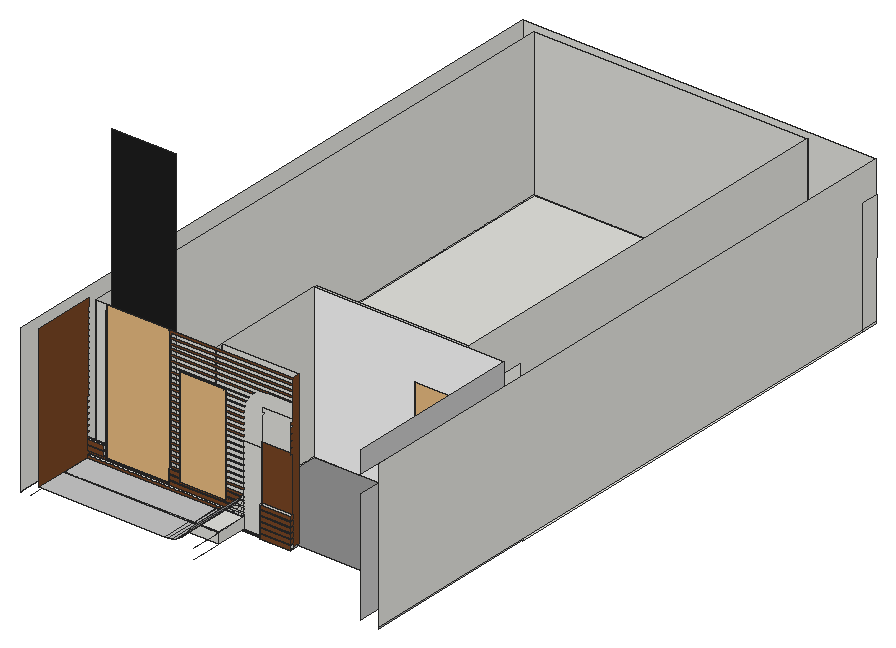
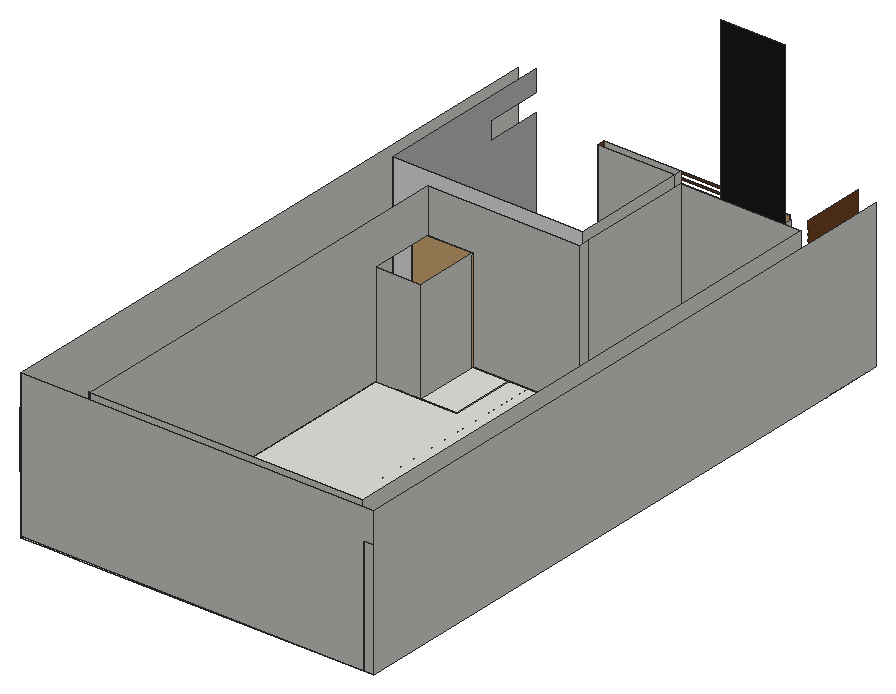
# SketchUp Ruby script. Lengths in inches.
U = 1.inch
M = Sketchup.active_model
def pt(a) = Geom::Point3d.new(a.map { |v| v * U })
def face(e, loops, mat)
  f = e.add_face(loops[0].map { |a| pt(a) })
  loops[1..].each { |l| e.add_face(l.map { |a| pt(a) }).erase! }
  f.material = f.back_material = mat if mat
  f
end
# faces: each face lists its corners as indices into pts; further lists are holes
def faces(e, pts, list, mat = nil) = list.each { |f| face(e, (f[0].is_a?(Array) ? f : [f]).map { |l| l.map { |i| pts[i] } }, mat) }
# xy, xz, yz: faces in a plane at the given z, y or x. An outline is a flat list of corners, or four numbers for a rectangle; further outlines are holes
def ring(l) = l.size == 4 ? [[l[0], l[1]], [l[2], l[1]], [l[2], l[3]], [l[0], l[3]]] : l.each_slice(2).to_a
def flat(e, list, mat, &to3) = list.each { |f| face(e, (f[0].is_a?(Array) ? f : [f]).map { |l| ring(l).map { |u, v| to3.(u, v) } }, mat) }
def xy(e, z, list, mat = nil) = flat(e, list, mat) { |x, y| [x, y, z] }
def xz(e, y, list, mat = nil) = flat(e, list, mat) { |x, z| [x, y, z] }
def yz(e, x, list, mat = nil) = flat(e, list, mat) { |y, z| [x, y, z] }
def lines(e, pts, list) = list.each { |a, b| e.add_line(pt(pts[a]), pt(pts[b])) }
# prism: a flat outline (further loops are holes) pulled along v
def prism(e, loops, v, mat = nil)
  f = face(e, loops, mat); d = Geom::Vector3d.new(v.map { |x| x * U })
  f.pushpull(f.normal.samedirection?(d) ? d.length : -d.length)
end
def box(e, o, s, mat = nil) = prism(e, [[o, [o[0] + s[0], o[1], o[2]], [o[0] + s[0], o[1] + s[1], o[2]], [o[0], o[1] + s[1], o[2]]]], [0, 0, s[2]], mat)
def at(x, y, z, deg = 0) = Geom::Transformation.translation(pt([x, y, z])) * Geom::Transformation.rotation(ORIGIN, Z_AXIS, deg.degrees)
def axes(o, x, y, z) = Geom::Transformation.new([*x, 0, *y, 0, *z, 0, *pt(o).to_a, 1])
def part(name) = M.definitions.add(name)
# library, detail: a bought-in or finely detailed component or shape, given as its bounding box
def library(name, o, s) = part(name).tap { |d| box(d.entities, o, s) }
def detail(e, o, s) = box(e.add_group.entities, o, s)
def put(e, d, t, mat = nil) = e.add_instance(d, t).tap { |i| i.material = mat if mat }
def group(e, t, mat = nil) = e.add_group.tap { |g| g.transformation = t; g.material = mat if mat }.entities
root = M.entities
M.materials.add("Moss 1").color = [97, 97, 43]
M.materials.add("[Color M00]").color = [255, 255, 255]
M.materials.add("[Color M02]").color = [198, 198, 198]
M.materials.add("[Color M03]").color = [170, 170, 170]
M.materials.add("[Color M04]1").color = [142, 142, 142]
M.materials.add("[Color M08]1").color = [30, 30, 30]
M.materials.add("[Groundcover_Wood_Mix]").color = [133, 121, 115]
M.materials.add("[Wood Veneer 01]").color = [120, 70, 37]
c1 = part("HCD  9x9 Indo Pot (Square)")
xy(c1.entities,0,[[0,0,9,9]])
xy(c1.entities,0.75,[[0.75,0.75,8.25,8.25]])
xy(c1.entities,7.52,[[0.75,0.75,8.25,8.25]],"Moss 1")
xy(c1.entities,9,[[[0,0,9,9],[0.75,0.75,8.25,8.25]]])
xz(c1.entities,0,[[0,0,9,9]])
xz(c1.entities,0.75,[[0.75,0.75,8.25,7.52],[0.75,7.52,8.25,9]])
xz(c1.entities,8.25,[[0.75,0.75,8.25,7.52],[0.75,7.52,8.25,9]])
xz(c1.entities,9,[[0,0,9,9]])
yz(c1.entities,0,[[0,0,9,9]])
yz(c1.entities,0.75,[[0.75,0.75,8.25,7.52],[0.75,7.52,8.25,9]])
yz(c1.entities,8.25,[[0.75,0.75,8.25,7.52],[0.75,7.52,8.25,9]])
yz(c1.entities,9,[[0,0,9,9]])
c2 = part("Group\#284")
detail(c2.entities,[0,0,0],[2.15,3.79,14.3])
c3 = part("Potted plant")
put(c3.entities,c1,axes([7.375,7.93,0],[1.35,0,0],[0,1.35,0],[0,0,1.35]))
g1 = group(c3.entities,at(34.01,16.59,10.48),"[Groundcover_Wood_Mix]")
put(g1,c2,axes([-21.39,-3.67,0.04],[1.0831,1.67432,0],[1.44561,-0.94233,-0.44822],[0.5095,-0.33212,1.35364]))
put(g1,c2,axes([-19.2,-0.0625,0.04],[0.06577,-1.58752,0],[-1.23,-0.01362,-0.59477],[-0.71488,-0.00792,0.95418]))
put(g1,c2,axes([-20.16,-2.02,1.03],[1.23757,0.97175,0],[0.71987,-0.88743,-0.73204],[0.35645,-0.43942,0.56976]))
put(g1,c2,axes([-20.43,-4.53,0.04],[0.02652,1.58591,0],[1.23087,-0.05659,-0.59477],[0.71539,-0.03289,0.95418]))
put(g1,c2,axes([-19.73,-2.8125,1.03],[-1.55944,0.41251,0],[0.26154,1.08365,-0.73204],[0.12951,0.53658,0.56976]))
put(g1,c2,axes([-19.27,-4.42,0.04],[-1.00701,1.78126,0],[1.48381,0.79245,-0.44822],[0.52297,0.2793,1.35364]))
put(g1,c2,axes([-17.53,-1.6,0.04],[-1.30559,-0.8818,0],[-0.71402,1.01403,-0.59477],[-0.41499,0.58936,0.95418]))
put(g1,c2,axes([-21.8,-1.55,0.04],[2.03404,-0.13573,0],[-0.064,-1.68745,-0.44822],[-0.02256,-0.59474,1.35364]))
put(g1,c2,axes([-19.33,-2.61,1.03],[-1.22683,-0.98484,0],[-0.72899,0.88019,-0.73204],[-0.36097,0.43583,0.56976]))
put(g1,c2,axes([-19.3,-2.11,1.03],[0.27974,-1.57083,0],[-1.11549,-0.16277,-0.73204],[-0.55235,-0.0806,0.56976]))
put(g1,c2,axes([-21.97,-3.02,0.04],[1.31205,0.87256,0],[0.70701,-1.01874,-0.59477],[0.41092,-0.59209,0.95418]))
put(g1,c2,axes([-17.81,-3.69,0.04],[-1.51859,0.55236,0],[0.39363,1.14324,-0.59477],[0.22878,0.66446,0.95418]))
put(g1,c2,axes([-20.2,-2.52,1.03],[-0.299,1.5679,0],[1.11299,0.17632,-0.73204],[0.55111,0.08731,0.56976]))
put(g1,c2,axes([-21.28,-0.49,0.04],[1.33266,-0.92103,0],[-0.68389,-0.99325,-0.59477],[-0.39748,-0.57728,0.95418]))
put(g1,c2,axes([-19.17,-0.27,0.04],[-0.5456,-1.92548,0],[1.93945,-0.59168,-0.26656],[0.28985,-0.08843,1.78359]))
put(g1,c2,axes([-17.96,-1.15,0.04],[-1.27123,-1.53638,0],[-1.33347,1.09526,-0.44822],[-0.46998,0.38602,1.35364]))
put(g1,c2,axes([-19.65,-1.83,1.03],[1.43123,-0.75657,0],[-0.50987,-0.98658,-0.73204],[-0.25247,-0.48851,0.56976]))
put(g1,c2,axes([-16.8,-2.55,0.04],[-1.5632,-0.30402,0],[0.34989,-1.54112,-0.20989],[0.05229,-0.23032,1.4044]))
put(g1,c2,axes([-21.84,-2.79,0.04],[1.97107,0.44464,0],[-0.50241,1.94504,-0.26656],[-0.07509,0.29069,1.78359]))
put(g1,c2,axes([-20.37,0.56,0.04],[0.7463,-1.42646,0],[1.4028,0.68931,-0.20989],[0.20965,0.10302,1.4044]))
put(g1,c2,axes([-17.99,-3.6,0.04],[-1.66024,1.21511,0],[-1.16467,-1.59132,-0.26656],[-0.17406,-0.23783,1.78359]))
put(g1,c2,axes([-21.54,-4.58,0.04],[0.59386,1.45638,0],[-1.47231,0.6251,-0.20989],[-0.22004,0.09342,1.4044]))
put(g1,c2,axes([-19.92,-0.17,0.04],[0.74111,-1.89898,0],[-1.5902,-0.56846,-0.44822],[-0.56047,-0.20035,1.35364]))
c4 = library("door (1)",[38.93,25.48,0],[40,9.94,82.68])
c5 = library("Group\#414",[0,0,0],[35.43,0.39,70.87])
xy(root,60.3,[[480.01,345.98,505.26,349.54]],"[Wood Veneer 01]")
xy(root,60.625,[[338.49,355.04,437.21,449.29],[441.95,355.04,480.01,449.29],[480.01,355.04,561.55,449.29],[338.49,449.29,338.49,804.16,480.01,804.16,480.01,458.23,437.21,458.23,437.21,449.29],[480.01,449.29,495.24,458.23],
  [543.24,449.29,568.49,449.29,568.49,811.1,480.01,811.1,480.01,804.16,561.55,804.16,561.55,458.23,543.24,458.23],[495.24,449.29,543.24,458.23],[480.01,458.23,495.24,458.23,495.24,511.73,543.24,511.73,543.24,458.23,561.55,458.23,561.55,804.16,480.01,804.16],[495.24,458.23,543.24,511.73],[495.24,458.23,543.24,511.73]])
xy(root,60.75,[[480.01,345.98,505.26,348.1]])
xy(root,61.72,[[338.58,322.42,338.63,348.1],[338.63,322.42,465.45,348.1]])
xy(root,61.75,[[612.67,301.92,612.67,348.42,612.66,348.42,612.66,449.29,574.17,449.29,574.17,458.23,568.49,458.23,568.49,811.1,612.68,811.1,612.68,301.92],[323.43,348.42,331.5,449.29],[331.5,348.42,331.55,449.29],[331.55,348.42,346.7,348.42,346.7,355.04,338.49,355.04,338.49,449.29,331.55,449.29],[346.7,348.42,441.95,348.42,441.95,449.29,437.21,449.29,437.21,355.04,346.7,355.04],
  [441.95,348.42,480.01,355.04],[480.01,348.42,505.26,355.04],[338.49,355.04,346.7,449.29],[346.7,355.04,437.21,449.29],[323.43,449.29,331.55,811.1],
  [338.49,449.29,437.21,449.29,437.21,458.23,495.24,458.23,495.24,511.73,561.55,511.73,561.55,804.16,338.49,804.16],[495.24,449.29,524.68,458.23],[524.68,449.29,574.17,458.23],[495.24,458.23,524.68,511.73],[524.68,458.23,543.24,511.73],
  [543.24,458.23,561.55,511.73],[561.55,458.23,562.67,804.16]])
xy(root,61.75,[[612.66,301.92,612.67,348.42],[480.01,346.79,505.26,348.42]],"[Color M03]")
xy(root,61.75,[[505.26,352.35,597.79,352.35,597.79,449.29,441.95,449.29,441.95,355.04,505.26,355.04]],"[Color M04]1")
xy(root,63.8,[[480.01,345.98,505.26,348.1]])
xy(root,65.14,[[480.01,345.98,505.26,348.1]],"[Wood Veneer 01]")
xy(root,68.1875,[[480.01,345.98,505.26,348.1]])
xy(root,69.52,[[480.01,345.98,505.26,348.1]],"[Wood Veneer 01]")
xy(root,70.22,[[441.44,322.42,465.45,348.1]])
xy(root,70.22,[[338.58,296.73,441.44,322.42]],"[Color M02]")
xy(root,70.42,[[444.57,322.42,465.45,348.1],[338.58,345.98,444.57,348.1]])
xy(root,70.42,[[338.58,322.42,444.57,345.98]],"[Color M02]")
xy(root,72.57,[[338.58,345.98,451.7,348.1],[480.01,345.98,505.26,348.1]])
xy(root,73.68,[[352.5,348.1,404.9375,354.42]])
xy(root,73.91,[[405.46,345.98,454.16,348.1]])
xy(root,73.91,[[480.01,345.98,505.26,348.1]],"[Wood Veneer 01]")
xy(root,75.875,[[338.58,345.98,352.5,348.1]])
xy(root,76.96,[[405.46,345.98,458.09,348.1],[480.01,345.98,505.26,348.1]])
xy(root,78.29,[[405.46,345.98,459.33,348.1],[480.01,345.98,505.26,348.1]])
xy(root,79.59,[[338.58,345.98,352.5,348.1]])
xy(root,80.25,[[338.58,345.98,352.5,348.1]])
xy(root,81.34,[[405.46,345.98,461.65,348.1],[480.01,345.98,505.26,348.1]])
xy(root,82.68,[[405.46,345.98,462.46,348.1],[480.01,345.98,505.26,348.1]])
xy(root,83.97,[[338.58,345.98,352.5,348.1]])
xz(root,322.42,[[338.58,61.72,465.45,70.22],[338.58,70.22,465.45,70.42]])
xz(root,345.98,[[419.16,81.34,450.71,82.68]])
xz(root,345.98,[[480.01,60.75,505.26,63.8],[480.01,65.14,505.26,68.1875],[480.01,69.52,505.26,72.57],[338.58,70.42,444.57,70.42,447.66,71.03,450.63,72.04,451.7,72.57,338.58,72.57],[405.46,73.91,454.16,73.91,456.06,75.18,458.09,76.96,405.46,76.96],
  [480.01,73.91,505.26,76.96],[338.58,75.875,352.5,79.59],[405.46,78.29,419.16,81.34],[419.16,78.29,450.71,81.34],[450.71,78.29,459.33,78.29,460.49,79.61,461.65,81.34,450.71,81.34],
  [480.01,78.29,505.26,81.34],[338.58,80.25,352.5,83.97],[405.46,82.68,419.16,85.73],[419.16,82.68,450.71,85.73],[450.71,82.68,462.46,82.68,463.625,85.04,463.86,85.73,450.71,85.73],
  [480.01,82.68,505.26,85.73]],"[Wood Veneer 01]")
xz(root,348.1,[[405.46,60.75,405.46,61.4,454.2,61.17,454.78,61.16,454.16,60.75],[454.16,60.75,454.78,61.16,459.68,61.14,459.33,60.75],[459.33,60.75,459.68,61.14,462.65,61.125,462.46,60.75],[462.46,60.75,462.65,61.125,464.4375,61.12,464.3125,60.75],[464.3125,60.75,464.4375,61.12,465.3,61.11,465.27,60.75],
  [465.27,60.75,465.3,61.11,465.45,61.11,465.45,60.75],[480.01,61.04,480.01,61.11,465.45,61.11],[465.3,61.11,465.3,61.17,464.45,61.17,464.4375,61.12],[465.3,61.11,465.45,61.17],[465.45,61.11,480.01,61.17],
  [464.4375,61.12,464.45,61.17,462.67,61.17,462.65,61.125],[462.65,61.125,462.67,61.17,459.7,61.17,459.68,61.14],[459.68,61.14,459.7,61.17,454.78,61.17,454.78,61.16],[454.78,61.16,454.78,61.17,454.2,61.17],[454.2,61.17,454.78,61.17,455.2,61.44,441.44,61.44,444.57,61.65,455.5,61.65,455.6,61.72,405.46,61.72,405.46,61.4],
  [454.78,61.17,459.7,61.17,459.94,61.44,460.125,61.65,460.18,61.72,455.6,61.72,455.2,61.44],[459.7,61.17,462.67,61.17,462.8,61.44,462.9,61.65,462.9375,61.72,460.18,61.72,460.125,61.65,459.94,61.44],[462.67,61.17,464.45,61.17,464.55,61.44,464.62,61.65,464.64,61.7,464.64,61.72,462.9375,61.72,462.9,61.65,462.8,61.44],[464.45,61.17,465.3,61.17,465.32,61.44,465.33,61.65,465.33,61.72,464.64,61.72,464.64,61.7,464.62,61.65,464.55,61.44],[465.3,61.17,465.45,61.17,465.45,61.72,465.33,61.72,465.33,61.65,465.32,61.44],
  [465.45,61.17,480.01,61.72],[405.46,61.4,405.46,61.72,338.63,61.72,346.76,61.68],[441.44,61.44,455.2,61.44,455.5,61.65,444.57,61.65],[338.58,61.72,405.46,61.72,405.46,63.8,465.45,63.8,465.45,65.14,405.46,65.14,405.46,68.1875,465.45,68.1875,465.45,69.52,405.46,69.52,338.58,70.42],[405.46,61.72,455.6,61.72,456.06,62.02,458.09,63.8,405.46,63.8],
  [455.6,61.72,460.18,61.72,460.49,62.07,461.65,63.8,458.09,63.8,456.06,62.02],[460.18,61.72,462.9375,61.72,463.625,63.11,463.86,63.8,461.65,63.8,460.49,62.07],[462.9375,61.72,464.64,61.72,465.05,63.8,463.86,63.8,463.625,63.11],[464.64,61.72,465.33,61.72,465.45,63.53,465.45,63.8,465.05,63.8],[465.33,61.72,465.45,61.72,465.45,63.53],
  [465.45,61.72,480.01,126.53],[405.46,65.14,464.3125,65.14,464.55,65.83,464.62,66.04,464.64,66.09,465.05,68.1875,405.46,68.1875],[464.3125,65.14,465.27,65.14,465.32,65.83,465.33,66.04,465.45,67.92,465.45,68.1875,465.05,68.1875,464.64,66.09,464.62,66.04,464.55,65.83],[465.27,65.14,465.45,65.14,465.45,67.92,465.33,66.04,465.32,65.83],[480.01,65.14,505.26,68.1875],
  [441.44,65.83,455.2,65.83,455.5,66.04,444.57,66.04],[405.46,69.52,454.16,69.52,455.2,70.22,441.44,70.22,444.57,70.42,338.58,70.42],[454.16,69.52,459.33,69.52,459.94,70.22,455.2,70.22],[459.33,69.52,462.46,69.52,462.8,70.22,459.94,70.22],[462.46,69.52,464.3125,69.52,464.55,70.22,462.8,70.22],
  [464.3125,69.52,465.27,69.52,465.32,70.22,464.55,70.22],[465.27,69.52,465.45,69.52,465.45,70.22,465.32,70.22],[480.01,69.52,505.26,72.57],[441.44,70.22,455.2,70.22,455.5,70.42,444.57,70.42],[455.2,70.22,455.5,70.42,460.125,70.42,459.94,70.22],
  [459.94,70.22,460.125,70.42,462.9,70.42,462.8,70.22],[462.8,70.22,462.9,70.42,464.62,70.42,464.55,70.22],[464.55,70.22,464.62,70.42,465.33,70.42,465.32,70.22],[465.32,70.22,465.33,70.42,465.45,70.42,465.45,70.22],[338.58,70.42,338.58,72.57,451.7,72.57,450.63,72.04,447.66,71.03,444.57,70.42],
  [444.57,70.42,455.5,70.42,456.06,70.79,458.09,72.57,451.7,72.57,450.63,72.04,447.66,71.03],[405.46,73.91,405.46,76.96,458.09,76.96,456.06,75.18,454.16,73.91],[454.16,73.91,459.33,73.91,460.49,75.23,461.65,76.96,458.09,76.96,456.06,75.18],[480.01,73.91,505.26,76.96],[338.58,75.875,352.5,79.59],
  [405.46,78.29,405.46,81.34,461.65,81.34,460.49,79.61,459.33,78.29],[459.33,78.29,462.46,78.29,463.625,80.65,463.86,81.34,461.65,81.34,460.49,79.61],[480.01,78.29,505.26,81.34],[338.58,79.59,352.5,80.25],[338.58,80.25,352.5,83.97],
  [405.46,82.68,405.46,85.73,463.86,85.73,463.625,85.04,462.46,82.68],[462.46,82.68,464.3125,82.68,464.64,83.63,465.05,85.73,463.86,85.73,463.625,85.04],[480.01,82.68,505.26,85.73],[338.58,83.97,352.5,84.625]])
xz(root,348.1,[[480.01,60.75,505.26,63.8],[338.58,72.57,451.7,72.57,453.45,73.43,454.16,73.91,405.46,73.91,405.46,76.96,458.09,76.96,458.42,77.25,459.33,78.29,405.46,78.29,405.46,81.34,461.65,81.34,462.24,82.22,462.46,82.68,405.46,82.68,405.46,85.73,463.86,85.73,464.3125,87.0625,405.46,87.0625,405.46,90.11,465.05,90.11,465.25,91.1,465.27,91.45,405.46,91.45,405.46,94.5,465.45,94.5,465.45,95.83,405.46,95.83,405.46,98.88,465.45,98.88,465.45,100.22,405.46,100.22,405.46,103.27,465.45,103.27,465.45,104.6,405.46,104.6,405.46,107.66,465.45,107.66,465.45,108.99,405.46,108.99,405.46,112.04,465.45,112.04,465.45,113.375,405.46,113.375,405.46,116.43,465.45,116.43,465.45,117.76,405.46,117.76,405.46,120.8125,465.45,120.8125,465.45,122.15,405.46,122.15,405.46,125.2,465.45,125.2,465.45,126.53,405.46,126.53,405.46,129.58,465.45,129.58,465.45,130.92,405.48,130.92,405.48,133.82,465.45,133.82,465.45,135.29,405.48,135.29,405.48,138.2,465.45,138.2,465.45,139.67,405.48,139.67,405.48,142.57,465.45,142.57,465.45,144.04,405.48,144.04,405.48,146.95,465.45,146.95,465.45,147.4,465.52,148.42,405.48,148.42,405.48,151.32,465.87,151.32,466.04,152.17,405.48,152.17,405.48,155.07,466.92,155.07,467.06,155.46,467.53,156.42,405.48,156.42,405.48,159.32,469.2,159.32,469.81,160.23,469.87,160.29,405.48,160.29,405.48,163.2,472.65,163.2,473.69,164.11,474.62,164.73,405.48,164.73,405.48,167.63,480.73,167.63,481.07,167.75,483.77,168.29,486.52,168.47,505.26,168.47,505.26,168.79,405.48,168.79,405.48,171.7,505.26,171.7,505.26,173.11,405.48,173.11,405.48,176.01,505.26,176.01,505.26,177.48,405.48,177.48,405.48,180.38,505.26,180.38,505.26,181.86,405.48,181.86,405.48,184.76,505.26,184.76,505.26,186.3125,404.9375,186.3125,404.9375,73.68,352.5,73.68,352.5,75.875,338.58,75.875]],"[Wood Veneer 01]")
xz(root,348.42,[[612.66,60.625,612.67,61.75],[480.01,61.04,480.01,61.75,346.7,61.75,346.7,61.68,346.76,61.68],[346.7,61.68,346.7,61.75,331.55,61.75,338.63,61.72],[323.43,61.75,323.43,61.79,331.5,61.75],[441.95,61.75,480.01,61.75,480.01,150.58,480.57,150.58,480.79,151.04,481.22,151.68,481.72,152.25,481.75,152.27,480.01,152.27,480.01,156.4,505.26,156.4,505.26,186.3125,441.95,186.3125]])
xz(root,348.42,[[480.01,61.75,505.26,130.59]],"[Wood Veneer 01]")
xz(root,354.42,[[352.5,73.68,404.9375,312.81]],"[Color M08]1")
xz(root,355.04,[[338.49,60.625,437.21,61.75],[441.95,60.625,480.01,61.75],[338.49,61.75,437.21,181.75],[441.95,61.75,505.26,186.3125]])
xz(root,449.29,[[612.66,60.41,597.79,60.48,586.74,60.54,568.49,60.625,612.66,60.625],[331.5,60.48,346.7,60.625],[346.7,60.48,346.7,60.625,568.49,60.625,586.74,60.54,597.79,60.48],[331.5,60.625,331.5,61.75,331.55,61.75,346.7,61.68,346.7,60.625],[346.7,60.625,437.21,61.75],
  [437.21,60.625,441.95,61.75],[441.95,60.625,495.24,61.75],[495.24,60.625,561.55,61.75],[561.55,60.625,612.66,61.75],[346.7,61.68,331.55,61.75,346.7,61.75]])
xz(root,449.29,[[441.95,61.75,524.68,61.75,524.68,145.75,574.17,145.75,574.17,61.75,597.79,61.75,597.79,186.3125,441.95,186.3125]],"[Color M00]")
xz(root,458.23,[[437.21,60.625,495.24,61.75],[495.24,60.625,543.24,61.75],[543.24,60.625,561.55,61.75],[437.21,61.75,437.21,181.75,561.55,181.75,561.55,145.75,574.17,145.75,574.17,61.75]])
xz(root,511.73,[[495.24,60.625,543.24,61.75],[524.68,61.75,561.55,145.75]])
xz(root,804.16,[[338.49,60.625,561.55,61.75],[338.49,61.75,561.55,181.75],[561.55,61.75,562.67,181.75]])
xz(root,811.1,[[323.43,61.75,323.43,156.98,332,156.9375,331.55,61.75],[331.55,61.75,332,156.9375,323.43,156.98,323.43,181.75,612.68,181.75,612.68,61.75]])
yz(root,323.43,[[296.73,61.75,348.42,61.79],[348.42,61.75,348.42,61.79,296.73,61.79,296.73,181.75,811.1,181.75,811.1,61.75]])
yz(root,338.49,[[355.04,60.625,804.16,61.75],[355.04,61.75,804.16,181.75]])
yz(root,338.58,[[322.42,61.72,348.1,61.75],[322.42,61.75,348.1,70.42],[345.98,70.42,348.1,72.57],[345.98,75.875,348.1,79.59],[345.98,80.25,348.1,83.97]])
yz(root,338.58,[[296.73,70.22,322.42,70.22,322.42,70.42,345.98,70.42,345.98,72.57,348.1,72.57,348.1,75.875,345.98,75.875,345.98,79.59,348.1,79.59,348.1,80.25,345.98,80.25,345.98,83.97,348.1,83.97,348.1,84.625,345.98,84.625,345.98,88.34,348.1,88.34,348.1,89,345.98,89,345.98,92.72,348.1,92.72,348.1,93.375,345.98,93.375,345.98,97.09,348.1,97.09,348.1,97.75,345.98,97.75,345.98,101.47,348.1,101.47,348.1,102.125,345.98,102.125,345.98,105.84,348.1,105.84,348.1,106.5,345.98,106.5,345.98,110.22,348.1,110.22,348.1,110.875,345.98,110.875,345.98,114.59,348.1,114.59,348.1,115.25,346.73,115.25,346.73,118.97,348.1,118.97,348.1,119.625,346.73,119.625,346.73,123.34,348.1,123.34,348.1,124,346.73,124,346.73,127.72,348.1,127.72,348.1,128.375,346.73,128.375,346.73,132.09,348.1,132.09,348.1,132.75,346.73,132.75,346.73,136.47,348.1,136.47,348.1,137.125,346.73,137.125,346.73,140.84,348.1,140.84,348.1,141.5,346.73,141.5,346.73,145.22,348.1,145.22,348.1,145.875,346.73,145.875,346.73,149.59,348.1,149.59,348.1,150.25,346.73,150.25,346.73,153.97,348.1,153.97,348.1,154.625,346.73,154.625,346.73,158.34,348.1,158.34,348.1,159,346.73,159,346.73,162.72,348.1,162.72,348.1,163.375,346.73,163.375,346.73,167.09,348.1,167.09,348.1,167.75,346.73,167.75,346.73,171.47,348.1,171.47,348.1,172.125,346.73,172.125,346.73,175.84,348.1,175.84,348.1,176.5,346.73,176.5,346.73,180.22,348.1,180.22,348.1,186.3125,296.73,186.3125]],"[Wood Veneer 01]")
yz(root,352.5,[[348.1,73.68,354.42,181.75],[345.98,75.875,348.1,76.75],[345.98,76.75,348.1,79.59],[345.98,80.25,348.1,81.125],[345.98,81.125,348.1,83.97]])
yz(root,404.9375,[[348.1,73.68,354.42,181.75]])
yz(root,405.46,[[345.98,73.91,348.1,76.96],[345.98,78.29,348.1,81.34],[345.98,82.68,348.1,85.73]])
yz(root,437.21,[[355.04,60.625,449.29,61.75],[449.29,60.625,458.23,61.75],[355.04,61.75,449.29,181.75],[449.29,61.75,458.23,181.75]])
yz(root,441.95,[[355.04,60.625,449.29,61.75],[348.42,61.75,355.04,186.3125],[355.04,61.75,449.29,186.3125]])
yz(root,465.45,[[322.42,61.72,348.1,70.22],[322.42,70.22,348.1,70.42]])
yz(root,480.01,[[348.1,60.625,348.42,61.04],[348.42,60.625,355.04,61.04],[355.04,60.625,811.1,61.04],[345.98,60.75,348.1,61.04],[345.98,61.04,346.79,61.11],
  [346.79,61.04,348.1,61.11],[348.1,61.04,348.42,61.11],[345.98,61.11,346.79,61.17],[346.79,61.11,348.1,61.17],[348.1,61.11,348.42,61.17],
  [345.98,61.17,346.79,61.72],[346.79,61.17,348.1,61.72],[348.1,61.17,348.42,61.72],[345.98,61.72,346.79,61.72,346.79,61.75,348.1,61.75,348.1,63.8,345.98,63.8],[346.79,61.72,348.1,61.75],
  [348.1,61.72,348.42,61.75],[348.1,61.75,348.42,130.59],[345.98,65.14,348.1,68.1875],[345.98,69.52,348.1,72.57],[345.98,73.91,348.1,76.96],
  [345.98,78.29,348.1,81.34],[345.98,82.68,348.1,85.73]])
yz(root,495.24,[[449.29,60.625,458.23,61.75],[458.23,60.625,511.73,61.75]])
yz(root,505.26,[[345.98,60.75,346.79,60.75,346.79,61.75,348.1,61.75,348.1,63.8,345.98,63.8],[346.79,60.75,348.1,61.75]])
yz(root,505.26,[[346.79,60.3,352.35,60.3,352.35,61.75,348.1,61.75,348.1,60.75,346.79,60.75]],"[Color M03]")
yz(root,505.26,[[348.42,61.75,355.04,61.75,355.04,186.3125,348.42,186.3125,348.42,153.97,346.17,153.97,346.17,152.27,348.42,152.27,348.42,150.58,345.98,150.58,345.98,146.46,348.42,146.46,348.42,145.21,345.98,145.21,345.98,141.08,348.42,141.08,348.42,139.85,345.98,139.85,345.98,135.72,348.42,135.72,348.42,134.72,345.98,134.72,345.98,130.59,348.42,130.59],[345.98,65.14,348.1,68.1875],[345.98,69.52,348.1,72.57],[345.98,73.91,348.1,76.96],[345.98,78.29,348.1,81.34],
  [345.98,82.68,348.1,85.73]],"[Wood Veneer 01]")
yz(root,524.68,[[449.29,61.75,511.73,145.75]])
yz(root,543.24,[[458.23,60.625,511.73,61.75]])
yz(root,561.55,[[458.23,60.625,804.16,61.75],[511.73,61.75,511.73,145.75,458.23,145.75,458.23,181.75,804.16,181.75,804.16,61.75]])
yz(root,574.17,[[449.29,61.75,458.23,145.75]])
yz(root,597.79,[[301.92,61.75,301.92,153.97,348.1,153.97,348.1,168.47,301.92,168.47,301.92,186.3125,449.29,186.3125,449.29,61.75]],"[Color M02]")
yz(root,612.66,[[348.42,60.625,449.29,61.75]])
yz(root,612.66,[[301.92,60.625,348.42,61.75]],"[Color M03]")
yz(root,612.68,[[301.92,61.75,811.1,181.75]])
p = [[586.74,811.1,60.54],[586.74,449.29,60.54],[597.79,449.29,60.48],[612.66,449.29,60.41],[612.67,449.29,60.41],[612.67,797.71,60.41],
  [612.67,811.1,60.41],[612.68,797.71,61.75],[612.68,811.1,61.75],[568.49,811.1,60.625],[568.49,449.29,60.625],[480.01,346.79,61.04],
  [480.01,348.1,61.04],[465.45,348.1,61.11],[465.3,348.1,61.11],[464.4375,348.1,61.12],[462.65,348.1,61.125],[459.68,348.1,61.14],
  [454.78,348.1,61.16],[454.2,348.1,61.17],[405.46,348.1,61.4],[346.76,348.1,61.68],[346.76,346.79,61.68],[346.76,348.42,61.68],
  [480.01,348.42,61.04],[346.76,811.1,61.68],[346.76,449.29,61.68],[480.01,355.04,61.04],[480.01,811.1,61.04],[338.63,322.42,61.72],
  [338.63,348.1,61.72],[338.58,348.1,61.72],[331.55,348.1,61.75],[323.43,348.1,61.79],[323.43,322.42,61.79],[331.55,322.42,61.75],
  [338.58,322.42,61.72],[338.63,348.42,61.72],[331.55,348.42,61.75],[331.5,348.42,61.75],[323.43,348.42,61.79],[331.55,449.29,61.75],
  [346.7,348.42,61.68],[346.7,449.29,61.68],[331.55,798.27,61.75],[331.55,811.1,61.75],[613.12,811.1,155.6],[613.12,797.71,155.6],
  [332,798.27,156.9375],[332,811.1,156.9375],[441.44,296.73,70.22],[444.57,296.73,70.42],[444.57,322.42,70.42],[444.57,345.98,70.42],
  [444.57,348.1,70.42],[441.44,348.1,70.22],[441.44,322.42,70.22],[447.66,296.73,71.03],[447.66,345.98,71.03],[447.66,348.1,71.03],
  [450.63,296.73,72.04],[450.63,345.98,72.04],[450.63,348.1,72.04],[453.45,296.73,73.43],[453.45,348.1,73.43],[451.7,348.1,72.57],
  [451.7,345.98,72.57],[456.06,296.73,75.18],[456.06,345.98,75.18],[454.16,345.98,73.91],[454.16,348.1,73.91],[456.06,348.1,75.18],
  [458.42,296.73,77.25],[458.42,348.1,77.25],[458.09,348.1,76.96],[458.09,345.98,76.96],[460.49,296.73,79.61],[460.49,345.98,79.61],
  [459.33,345.98,78.29],[459.33,348.1,78.29],[460.49,348.1,79.61],[462.24,296.73,82.22],[462.24,348.1,82.22],[461.65,348.1,81.34],
  [461.65,345.98,81.34],[463.625,296.73,85.04],[463.625,345.98,85.04],[462.46,345.98,82.68],[462.46,348.1,82.68],[463.625,348.1,85.04],
  [561.55,355.04,61.75],[561.55,355.04,60.625],[465.45,322.42,61.72],[465.45,296.73,61.72],[465.45,296.73,70.22],[465.45,322.42,70.22],
  [331.55,296.73,61.75],[465.45,348.1,82.68],[465.27,348.1,82.68],[465.45,348.1,85.46],[464.3125,348.1,82.68],[463.86,348.1,81.34],
  [465.05,348.1,81.34],[465.27,348.1,78.29],[465.45,348.1,81.07],[465.45,348.1,78.29],[464.3125,348.1,78.29],[464.64,348.1,79.24],
  [465.45,348.1,81.34],[462.46,348.1,78.29],[465.05,348.1,76.96],[465.45,348.1,76.96],[464.64,348.1,74.86],[464.3125,348.1,73.91],
  [465.27,348.1,73.91],[465.45,348.1,76.6875],[462.46,348.1,73.91],[459.33,348.1,73.91],[463.86,348.1,76.96],[463.625,348.1,76.27],
  [465.45,348.1,73.91],[461.65,348.1,76.96],[460.49,348.1,70.84],[461.65,348.1,72.57],[463.86,348.1,72.57],[465.05,348.1,72.57],
  [464.64,348.1,70.47],[465.45,348.1,72.57],[463.625,348.1,71.88],[458.09,348.1,72.57],[460.125,348.1,70.42],[464.62,348.1,70.42],
  [465.33,348.1,70.42],[465.45,348.1,72.3],[462.9,348.1,70.42],[460.125,348.1,66.04],[460.49,348.1,66.45],[459.94,348.1,65.83],
  [461.65,348.1,68.1875],[462.46,348.1,65.14],[462.8,348.1,65.83],[459.33,348.1,65.14],[455.5,348.1,66.04],[456.06,348.1,66.41],
  [458.09,348.1,68.1875],[454.16,348.1,65.14],[455.2,348.1,65.83],[463.625,348.1,67.5],[463.86,348.1,68.1875],[462.9,348.1,66.04]]
faces(root,p,[[0,1,2,3,4,5,6],[5,7,8,6],[9,10,1,0],[25,26,23,24,27,28],[29,30,31,32,33,34,35,36],[30,37,38,39,40,33,32,31],[41,38,37,42,23,26,43],[44,41,43,26,25,45],
  [46,8,7,47],[48,44,45,49],[59,54,53,58],[62,59,58,61],[65,62,61,66],[71,70,69,68],[74,71,68,75],[80,79,78,77],
  [83,80,77,84],[89,88,87,86]])
faces(root,p,[[11,12,13,14,15,16,17,18,19,20,21,22],[23,21,20,19,18,17,16,15,14,13,12,24]],"[Color M03]")
faces(root,p,[[50,51,52,53,54,55,56],[51,57,58,53,52],[57,60,61,58],[60,63,64,65,66,61],[63,67,68,69,70,64],[67,72,73,74,75,68],[72,76,77,78,79,73],[76,81,82,83,84,77],
  [81,85,86,87,88,82]],"[Color M02]")
lines(root,p,[[90,91],[92,93],[94,95],[38,32],[35,96],[32,35],[97,98],[98,99],[98,100],[101,102],[103,104],[105,103],
  [106,107],[107,102],[102,108],[106,109],[103,106],[110,111],[112,110],[113,112],[114,115],[114,113],[116,117],[118,110],
  [116,119],[119,118],[120,114],[113,116],[121,118],[122,123],[124,125],[126,125],[125,127],[123,124],[128,124],[129,123],
  [130,122],[131,126],[132,133],[134,128],[135,136],[137,135],[136,138],[139,140],[141,137],[142,143],[143,144],[145,146],
  [147,148],[140,149],[149,147]])
put(root,c3,axes([570.9375,409.59,61.75],[1.19,0,0],[0,1.19,0],[0,0,1.19]))
put(root,c4,axes([476.51,423.81,61.75],[1.23732,0,0],[0,1,0],[0,0,1.016]))
put(root,c5,axes([352.5,348.59,73.68],[1.4799,0,0],[0,1.58558,0],[0,0,1.58558]),"[Color M00]")
put(root,c5,axes([414.99,345.53,79.39],[1.06553,0,0],[0,1.14162,0],[0,0,1.14162]),"[Color M00]")
